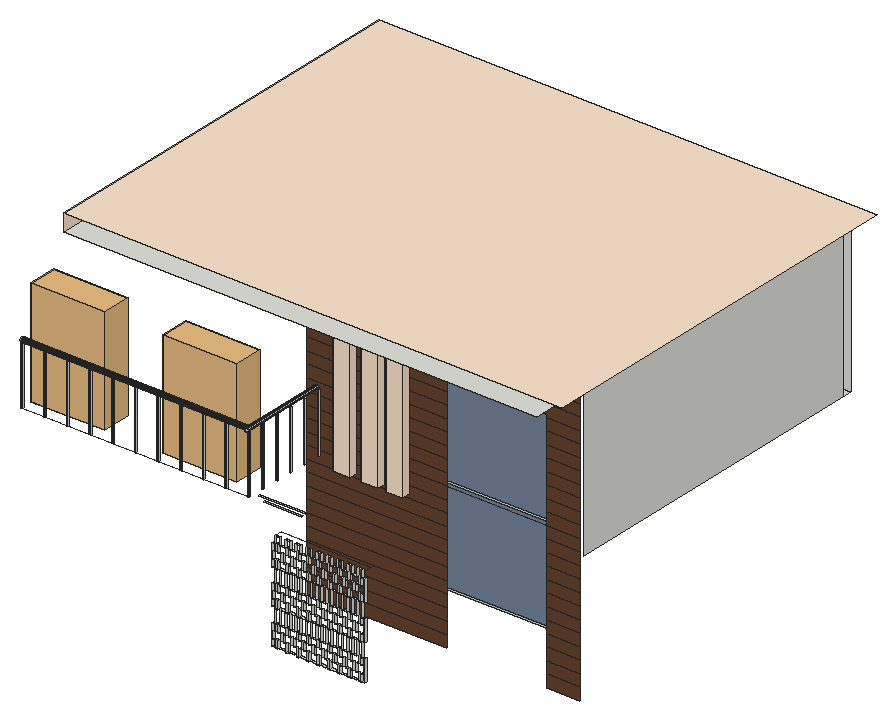
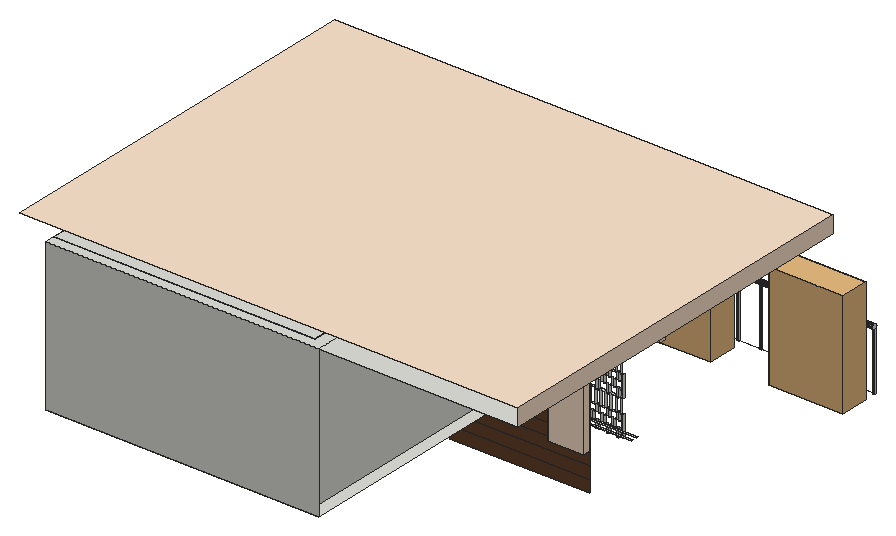
# SketchUp Ruby script. Lengths in inches.
U = 1.inch
M = Sketchup.active_model
def pt(a) = Geom::Point3d.new(a.map { |v| v * U })
def face(e, loops, mat)
  f = e.add_face(loops[0].map { |a| pt(a) })
  loops[1..].each { |l| e.add_face(l.map { |a| pt(a) }).erase! }
  f.material = f.back_material = mat if mat
  f
end
# faces: each face lists its corners as indices into pts; further lists are holes
def faces(e, pts, list, mat = nil) = list.each { |f| face(e, (f[0].is_a?(Array) ? f : [f]).map { |l| l.map { |i| pts[i] } }, mat) }
# xy, xz, yz: faces in a plane at the given z, y or x. An outline is a flat list of corners, or four numbers for a rectangle; further outlines are holes
def ring(l) = l.size == 4 ? [[l[0], l[1]], [l[2], l[1]], [l[2], l[3]], [l[0], l[3]]] : l.each_slice(2).to_a
def flat(e, list, mat, &to3) = list.each { |f| face(e, (f[0].is_a?(Array) ? f : [f]).map { |l| ring(l).map { |u, v| to3.(u, v) } }, mat) }
def xy(e, z, list, mat = nil) = flat(e, list, mat) { |x, y| [x, y, z] }
def xz(e, y, list, mat = nil) = flat(e, list, mat) { |x, z| [x, y, z] }
def yz(e, x, list, mat = nil) = flat(e, list, mat) { |y, z| [x, y, z] }
def lines(e, pts, list) = list.each { |a, b| e.add_line(pt(pts[a]), pt(pts[b])) }
# prism: a flat outline (further loops are holes) pulled along v
def prism(e, loops, v, mat = nil)
  f = face(e, loops, mat); d = Geom::Vector3d.new(v.map { |x| x * U })
  f.pushpull(f.normal.samedirection?(d) ? d.length : -d.length)
end
def box(e, o, s, mat = nil) = prism(e, [[o, [o[0] + s[0], o[1], o[2]], [o[0] + s[0], o[1] + s[1], o[2]], [o[0], o[1] + s[1], o[2]]]], [0, 0, s[2]], mat)
def at(x, y, z, deg = 0) = Geom::Transformation.translation(pt([x, y, z])) * Geom::Transformation.rotation(ORIGIN, Z_AXIS, deg.degrees)
def axes(o, x, y, z) = Geom::Transformation.new([*x, 0, *y, 0, *z, 0, *pt(o).to_a, 1])
def part(name) = M.definitions.add(name)
# library, detail: a bought-in or finely detailed component or shape, given as its bounding box
def library(name, o, s) = part(name).tap { |d| box(d.entities, o, s) }
def detail(e, o, s) = box(e.add_group.entities, o, s)
def put(e, d, t, mat = nil) = e.add_instance(d, t).tap { |i| i.material = mat if mat }
def group(e, t, mat = nil) = e.add_group.tap { |g| g.transformation = t; g.material = mat if mat }.entities
root = M.entities
M.materials.add("C01_Vanilla_Cream").color = [255, 230, 206]
M.materials.add("Glass_Mirror_01").color = [119, 135, 160]
M.materials.add("Wood_Veneer_15_1K").color = [103, 69, 45]
c1 = library("Group_2",[-1.28,-0.39,0],[21.22,20.51,48.44])
xy(root,373.98,[[283.14,137.21,284.89,138.74],[290.55,137.21,292.3,138.74],[297.96,137.21,299.71,138.74],[305.37,137.21,307.12,138.74],[312.78,137.21,314.53,138.74],
  [320.1875,137.21,321.94,138.74],[327.6,137.21,329.35,138.74],[335.01,137.21,336.76,138.74],[342.42,137.21,344.17,138.74]])
xy(root,374.38,[[280.31,137.21,282.27,138.74],[285.76,137.21,289.68,138.74],[293.17,137.21,297.09,138.74],[300.58,137.21,304.5,138.74],[307.99,137.21,311.91,138.74],
  [315.4,137.21,319.32,138.74],[322.81,137.21,326.73,138.74],[330.22,137.21,334.14,138.74],[337.63,137.21,341.55,138.74],[345.04,137.21,347,138.74]])
xy(root,379.25,[[281.18,137.21,283.14,138.74],[284.89,137.21,286.85,138.74],[288.59,137.21,290.55,138.74],[292.3,137.21,294.26,138.74],[296,137.21,297.96,138.74],
  [299.71,137.21,301.67,138.74],[303.41,137.21,305.37,138.74],[307.12,137.21,309.08,138.74],[310.82,137.21,312.78,138.74],[314.53,137.21,316.49,138.74],
  [318.23,137.21,320.1875,138.74],[321.94,137.21,323.9,138.74],[325.64,137.21,327.6,138.74],[329.35,137.21,331.31,138.74],[333.05,137.21,335.01,138.74],
  [336.76,137.21,338.72,138.74],[340.46,137.21,342.42,138.74],[344.17,137.21,346.13,138.74]])
xy(root,384.61,[[281.18,137.21,283.14,138.74],[284.89,137.21,286.85,138.74],[288.59,137.21,290.55,138.74],[292.3,137.21,294.26,138.74],[296,137.21,297.96,138.74],
  [299.71,137.21,301.67,138.74],[303.41,137.21,305.37,138.74],[307.12,137.21,309.08,138.74],[310.82,137.21,312.78,138.74],[314.53,137.21,316.49,138.74],
  [318.23,137.21,320.1875,138.74],[321.94,137.21,323.9,138.74],[325.64,137.21,327.6,138.74],[329.35,137.21,331.31,138.74],[333.05,137.21,335.01,138.74],
  [336.76,137.21,338.72,138.74],[340.46,137.21,342.42,138.74],[344.17,137.21,346.13,138.74]])
xy(root,389.47,[[280.31,137.21,282.27,138.74],[285.76,137.21,289.68,138.74],[293.17,137.21,297.09,138.74],[300.58,137.21,304.5,138.74],[307.99,137.21,311.91,138.74],
  [315.4,137.21,319.32,138.74],[322.81,137.21,326.73,138.74],[330.22,137.21,334.14,138.74],[337.63,137.21,341.55,138.74],[345.04,137.21,347,138.74]])
xy(root,389.875,[[283.14,137.21,284.89,138.74],[290.55,137.21,292.3,138.74],[297.96,137.21,299.71,138.74],[305.37,137.21,307.12,138.74],[312.78,137.21,314.53,138.74],
  [320.1875,137.21,321.94,138.74],[327.6,137.21,329.35,138.74],[335.01,137.21,336.76,138.74],[342.42,137.21,344.17,138.74]])
xy(root,399.61,[[283.14,137.21,284.89,138.74],[290.55,137.21,292.3,138.74],[297.96,137.21,299.71,138.74],[305.37,137.21,307.12,138.74],[312.78,137.21,314.53,138.74],
  [320.1875,137.21,321.94,138.74],[327.6,137.21,329.35,138.74],[335.01,137.21,336.76,138.74],[342.42,137.21,344.17,138.74]])
xy(root,400.01,[[280.31,137.21,282.27,138.74],[285.76,137.21,289.68,138.74],[293.17,137.21,297.09,138.74],[300.58,137.21,304.5,138.74],[307.99,137.21,311.91,138.74],
  [315.4,137.21,319.32,138.74],[322.81,137.21,326.73,138.74],[330.22,137.21,334.14,138.74],[337.63,137.21,341.55,138.74],[345.04,137.21,347,138.74]])
xy(root,404.88,[[281.18,137.21,283.14,138.74],[284.89,137.21,286.85,138.74],[288.59,137.21,290.55,138.74],[292.3,137.21,294.26,138.74],[296,137.21,297.96,138.74],
  [299.71,137.21,301.67,138.74],[303.41,137.21,305.37,138.74],[307.12,137.21,309.08,138.74],[310.82,137.21,312.78,138.74],[314.53,137.21,316.49,138.74],
  [318.23,137.21,320.1875,138.74],[321.94,137.21,323.9,138.74],[325.64,137.21,327.6,138.74],[329.35,137.21,331.31,138.74],[333.05,137.21,335.01,138.74],
  [336.76,137.21,338.72,138.74],[340.46,137.21,342.42,138.74],[344.17,137.21,346.13,138.74]])
xy(root,410.24,[[281.18,137.21,283.14,138.74],[284.89,137.21,286.85,138.74],[288.59,137.21,290.55,138.74],[292.3,137.21,294.26,138.74],[296,137.21,297.96,138.74],
  [299.71,137.21,301.67,138.74],[303.41,137.21,305.37,138.74],[307.12,137.21,309.08,138.74],[310.82,137.21,312.78,138.74],[314.53,137.21,316.49,138.74],
  [318.23,137.21,320.1875,138.74],[321.94,137.21,323.9,138.74],[325.64,137.21,327.6,138.74],[329.35,137.21,331.31,138.74],[333.05,137.21,335.01,138.74],
  [336.76,137.21,338.72,138.74],[340.46,137.21,342.42,138.74],[344.17,137.21,346.13,138.74]])
xy(root,415.1,[[280.31,137.21,282.27,138.74],[285.76,137.21,289.68,138.74],[293.17,137.21,297.09,138.74],[300.58,137.21,304.5,138.74],[307.99,137.21,311.91,138.74],
  [315.4,137.21,319.32,138.74],[322.81,137.21,326.73,138.74],[330.22,137.21,334.14,138.74],[337.63,137.21,341.55,138.74],[345.04,137.21,347,138.74]])
xy(root,415.5,[[283.14,137.21,284.89,138.74],[290.55,137.21,292.3,138.74],[297.96,137.21,299.71,138.74],[305.37,137.21,307.12,138.74],[312.78,137.21,314.53,138.74],
  [320.1875,137.21,321.94,138.74],[327.6,137.21,329.35,138.74],[335.01,137.21,336.76,138.74],[342.42,137.21,344.17,138.74]])
xy(root,425.24,[[283.14,137.21,284.89,138.74],[290.55,137.21,292.3,138.74],[297.96,137.21,299.71,138.74],[305.37,137.21,307.12,138.74],[312.78,137.21,314.53,138.74],
  [320.1875,137.21,321.94,138.74],[327.6,137.21,329.35,138.74],[335.01,137.21,336.76,138.74],[342.42,137.21,344.17,138.74]])
xy(root,425.64,[[280.31,137.21,282.27,138.74],[285.76,137.21,289.68,138.74],[293.17,137.21,297.09,138.74],[300.58,137.21,304.5,138.74],[307.99,137.21,311.91,138.74],
  [315.4,137.21,319.32,138.74],[322.81,137.21,326.73,138.74],[330.22,137.21,334.14,138.74],[337.63,137.21,341.55,138.74],[345.04,137.21,347,138.74]])
xy(root,430.51,[[281.18,137.21,283.14,138.74],[284.89,137.21,286.85,138.74],[288.59,137.21,290.55,138.74],[292.3,137.21,294.26,138.74],[296,137.21,297.96,138.74],
  [299.71,137.21,301.67,138.74],[303.41,137.21,305.37,138.74],[307.12,137.21,309.08,138.74],[310.82,137.21,312.78,138.74],[314.53,137.21,316.49,138.74],
  [318.23,137.21,320.1875,138.74],[321.94,137.21,323.9,138.74],[325.64,137.21,327.6,138.74],[329.35,137.21,331.31,138.74],[333.05,137.21,335.01,138.74],
  [336.76,137.21,338.72,138.74],[340.46,137.21,342.42,138.74],[344.17,137.21,346.13,138.74]])
xy(root,435.86,[[281.18,137.21,283.14,138.74],[284.89,137.21,286.85,138.74],[288.59,137.21,290.55,138.74],[292.3,137.21,294.26,138.74],[296,137.21,297.96,138.74],
  [299.71,137.21,301.67,138.74],[303.41,137.21,305.37,138.74],[307.12,137.21,309.08,138.74],[310.82,137.21,312.78,138.74],[314.53,137.21,316.49,138.74],
  [318.23,137.21,320.1875,138.74],[321.94,137.21,323.9,138.74],[325.64,137.21,327.6,138.74],[329.35,137.21,331.31,138.74],[333.05,137.21,335.01,138.74],
  [336.76,137.21,338.72,138.74],[340.46,137.21,342.42,138.74],[344.17,137.21,346.13,138.74]])
xy(root,440.73,[[280.31,137.21,282.27,138.74],[285.76,137.21,289.68,138.74],[293.17,137.21,297.09,138.74],[300.58,137.21,304.5,138.74],[307.99,137.21,311.91,138.74],
  [315.4,137.21,319.32,138.74],[322.81,137.21,326.73,138.74],[330.22,137.21,334.14,138.74],[337.63,137.21,341.55,138.74],[345.04,137.21,347,138.74]])
xy(root,441.13,[[283.14,137.21,284.89,138.74],[290.55,137.21,292.3,138.74],[297.96,137.21,299.71,138.74],[305.37,137.21,307.12,138.74],[312.78,137.21,314.53,138.74],
  [320.1875,137.21,321.94,138.74],[327.6,137.21,329.35,138.74],[335.01,137.21,336.76,138.74],[342.42,137.21,344.17,138.74]])
xy(root,446,[[282.27,137.21,285.76,138.74],[289.68,137.21,293.17,138.74],[297.09,137.21,300.58,138.74],[304.5,137.21,307.99,138.74],[311.91,137.21,315.4,138.74],
  [319.32,137.21,322.81,138.74],[326.73,137.21,330.22,138.74],[334.14,137.21,337.63,138.74],[341.55,137.21,345.04,138.74]])
xy(root,465,[[263.64,136.51,264.8,137.09],[282.61,189.3,294.64,194.88],[302.46,189.3,314.49,194.88],[320.42,189.3,332.45,194.88],[256.9,201,256.9,441,453,441,453,433.71,265.5,433.71,265.5,201],
  [185.32,287.91,211.07,293.09]])
xy(root,507.13,[[263.64,136.51,264.8,137.09]])
xy(root,549,[[357,198,429,199.5]])
xy(root,555.9375,[[130.74,287.91,185.32,293.09],[211.07,287.91,256.9,293.09]],"C01_Vanilla_Cream")
xy(root,573,[[[114,158.82,114,441,256.9,441,256.9,198,453,198,453,158.82],[320.42,189.3,332.45,194.88],[302.46,189.3,314.49,194.88],[282.61,189.3,294.64,194.88]],[256.9,198,256.9,441,453,441,453,433.71,265.5,433.71,265.5,201,453,201,453,198],[265.5,201,453,433.71]])
xy(root,579.87,[[130.74,287.91,256.9,293.09]])
xy(root,585,[[114,158.82,471,441]],"C01_Vanilla_Cream")
xz(root,135.29,[[263.64,507.13,264.01,507.18,264.36,507.32,264.66,507.55,264.89,507.85,265.04,508.2,265.09,508.58,265.04,508.96,264.89,509.31,264.66,509.61,264.36,509.84,264.01,509.98,263.64,510.03,263.26,509.98,262.91,509.84,262.61,509.61,262.38,509.31,262.27,509.05,262.24,508.96,262.1875,508.58,262.24,508.2,262.38,507.85,262.61,507.55,262.91,507.32,263.26,507.18]])
xz(root,136.51,[[100.9,465,102.07,507.13],[117.18,465,118.34,507.13],[133.45,465,134.62,507.13],[149.72,465,150.89,507.13],[166,465,167.16,507.13],
  [182.27,465,183.44,507.13],[198.54,465,199.71,507.13],[214.82,465,215.98,507.13],[231.09,465,232.26,507.13],[247.36,465,248.53,507.13],
  [263.64,465,264.8,507.13]])
xz(root,137.09,[[100.9,465,102.07,507.13],[117.18,465,118.34,507.13],[133.45,465,134.62,507.13],[149.72,465,150.89,507.13],[166,465,167.16,507.13],
  [182.27,465,183.44,507.13],[198.54,465,199.71,507.13],[214.82,465,215.98,507.13],[231.09,465,232.26,507.13],[247.36,465,248.53,507.13],
  [263.64,465,264.8,507.13]])
xz(root,148.6875,[[263.9,465,265.0625,507.13]])
xz(root,149.27,[[263.9,465,265.0625,507.13]])
xz(root,160.87,[[264.16,465,265.32,507.13]])
xz(root,161.46,[[264.16,465,265.32,507.13]])
xz(root,173.05,[[264.42,465,265.59,507.13]])
xz(root,173.64,[[264.42,465,265.59,507.13]])
xz(root,185.23,[[264.68,465,265.85,507.13]])
xz(root,185.82,[[264.68,465,265.85,507.13]])
xz(root,189.3,[[282.61,465,294.64,573],[302.46,465,314.49,573],[320.42,465,332.45,573]],"C01_Vanilla_Cream")
xz(root,194.88,[[282.61,465,294.64,573],[302.46,465,314.49,573],[320.42,465,332.45,573]])
xz(root,197.41,[[264.94,465,266.11,507.13]])
xz(root,198,[[264.94,494.88,266.11,503.56]])
xz(root,198,[[256.9,373.36,357,382.04],[429,373.36,453,382.04],[256.9,382.04,357,390.72],[429,382.04,453,390.72],[256.9,390.72,357,399.4],
  [429,390.72,453,399.4],[256.9,399.4,357,408.08],[429,399.4,453,408.08],[256.9,408.08,357,416.76],[429,408.08,453,416.76],
  [256.9,416.76,357,425.44],[429,416.76,453,425.44],[256.9,425.44,357,434.12],[429,425.44,453,434.12],[256.9,434.12,357,442.8],
  [429,434.12,453,442.8],[256.9,442.8,357,451.48],[429,442.8,453,451.48],[256.9,451.48,357,460.16],[429,451.48,453,460.16],
  [256.9,460.16,357,460.16,357,468.84,266.11,468.84,266.11,465,264.94,465,264.94,468.84,256.9,468.84],[429,460.16,453,468.84],[264.94,465,266.11,468.84],[256.9,468.84,264.94,477.52],[264.94,468.84,266.11,477.52],
  [266.11,468.84,357,477.52],[429,468.84,453,477.52],[256.9,477.52,264.94,486.2],[264.94,477.52,266.11,486.2],[266.11,477.52,357,486.2],
  [429,477.52,453,486.2],[256.9,486.2,264.94,494.88],[264.94,486.2,266.11,494.88],[266.11,486.2,357,494.88],[429,486.2,453,494.88],
  [256.9,494.88,264.94,503.56],[266.11,494.88,357,503.56],[429,494.88,453,503.56],[[256.9,503.56,264.94,503.56,264.94,507.13,266.11,507.13,266.11,503.56,357,503.56,357,512.24,256.9,512.24],[263.64,507.13,263.26,507.18,262.91,507.32,262.61,507.55,262.38,507.85,262.24,508.2,262.1875,508.58,262.24,508.96,262.38,509.31,262.61,509.61,262.91,509.84,263.26,509.98,263.64,510.03,264.01,509.98,264.36,509.84,264.66,509.61,264.89,509.31,265.04,508.96,265.09,508.58,265.04,508.2,264.89,507.85,264.66,507.55,264.36,507.32,264.01,507.18]],[264.94,503.56,266.11,507.13],
  [429,503.56,453,512.24],[256.9,512.24,357,520.92],[429,512.24,453,520.92],[256.9,520.92,357,529.6],[429,520.92,453,529.6],
  [256.9,529.6,357,538.28],[429,529.6,453,538.28],[256.9,538.28,357,546.96],[429,538.28,453,546.96],[256.9,546.96,357,546.96,357,549,429,549,429,546.96,453,546.96,453,555.64,256.9,555.64],
  [256.9,555.64,453,564.32],[256.9,564.32,453,573]],"Wood_Veneer_15_1K")
xz(root,199.5,[[357,410.35,429,411.35],[357,479.17,429,480.17],[357,548,429,549]])
xz(root,199.5,[[357,411.35,429,479.17],[357,480.17,429,548]],"Glass_Mirror_01")
xz(root,287.91,[[185.32,465,211.07,465,211.07,555.9375,256.9,555.9375,256.9,579.87,130.74,579.87,130.74,555.9375,185.32,555.9375]],"C01_Vanilla_Cream")
xz(root,293.09,[[185.32,465,185.32,555.9375,130.74,555.9375,130.74,579.87,256.9,579.87,256.9,555.9375,211.07,555.9375,211.07,465]],"C01_Vanilla_Cream")
xz(root,433.71,[[265.5,465,453,573]])
xz(root,441,[[256.9,465,453,573]])
yz(root,100.9,[[136.51,465,137.09,507.13],[137.24,507.1,137.09,507.13,136.86,507.17,136.51,507.34,136.22,507.6,136,507.91,135.875,508.28,135.85,508.67,135.92,509.05,136.09,509.39,136.34,509.6875,136.66,509.9,137.03,510.03,137.41,510.06,137.79,509.99,138.14,509.82,138.43,509.56,138.65,509.24,138.78,508.88,138.8,508.49,138.73,508.11,138.5625,507.77,138.3125,507.47,137.99,507.26,137.625,507.13]])
yz(root,102.07,[[136.51,465,137.09,507.13]])
yz(root,114,[[158.82,573,441,585]],"C01_Vanilla_Cream")
yz(root,117.18,[[136.51,465,137.09,507.13]])
yz(root,118.34,[[136.51,465,137.09,507.13]])
yz(root,130.74,[[287.91,555.9375,293.09,579.87]],"C01_Vanilla_Cream")
yz(root,133.45,[[136.51,465,137.09,507.13]])
yz(root,134.62,[[136.51,465,137.09,507.13]])
yz(root,149.72,[[136.51,465,137.09,507.13]])
yz(root,150.89,[[136.51,465,137.09,507.13]])
yz(root,166,[[136.51,465,137.09,507.13]])
yz(root,167.16,[[136.51,465,137.09,507.13]])
yz(root,182.27,[[136.51,465,137.09,507.13]])
yz(root,183.44,[[136.51,465,137.09,507.13]])
yz(root,185.32,[[287.91,465,293.09,555.9375]],"C01_Vanilla_Cream")
yz(root,198.54,[[136.51,465,137.09,507.13]])
yz(root,199.71,[[136.51,465,137.09,507.13]])
yz(root,211.07,[[287.91,465,293.09,555.9375]],"C01_Vanilla_Cream")
yz(root,214.82,[[136.51,465,137.09,507.13]])
yz(root,215.98,[[136.51,465,137.09,507.13]])
yz(root,231.09,[[136.51,465,137.09,507.13]])
yz(root,232.26,[[136.51,465,137.09,507.13]])
yz(root,247.36,[[136.51,465,137.09,507.13]])
yz(root,248.53,[[136.51,465,137.09,507.13]])
yz(root,256.9,[[287.91,555.9375,293.09,573],[287.91,573,293.09,579.87]])
yz(root,263.64,[[136.51,465,137.09,507.13],[137.24,507.1,137.625,507.13,137.09,507.13],[137.09,507.13,137.625,507.13,137.99,507.26,138.3125,507.47,138.5625,507.77,138.73,508.11,138.8,508.49,138.8,508.58,138.78,508.88,138.65,509.24,138.43,509.56,138.14,509.82,137.79,509.99,137.56,510.03,137.03,510.03,136.66,509.9,136.34,509.6875,136.09,509.39,135.92,509.05,135.85,508.67,135.875,508.28,136,507.91,136.22,507.6,136.51,507.34,136.86,507.17],[137.03,510.03,137.56,510.03,137.41,510.06]])
yz(root,263.9,[[148.6875,465,149.27,507.13]])
yz(root,264.16,[[160.87,465,161.46,507.13]])
yz(root,264.42,[[173.05,465,173.64,507.13]])
yz(root,264.68,[[185.23,465,185.82,507.13]])
yz(root,264.8,[[136.51,465,137.09,507.13]])
yz(root,264.94,[[197.41,465,198,507.13]])
yz(root,265.0625,[[148.6875,465,149.27,507.13]])
yz(root,265.32,[[160.87,465,161.46,507.13]])
yz(root,265.5,[[201,465,433.71,573]])
yz(root,265.59,[[173.05,465,173.64,507.13]])
yz(root,265.85,[[185.23,465,185.82,507.13]])
yz(root,266.11,[[197.41,465,198,507.13]])
yz(root,280.31,[[137.21,374.38,138.74,389.47],[137.21,400.01,138.74,415.1],[137.21,425.64,138.74,440.73]])
yz(root,281.18,[[137.21,379.25,138.74,384.61],[137.21,404.88,138.74,410.24],[137.21,430.51,138.74,435.86]])
yz(root,282.27,[[137.21,389.47,138.74,400.01],[137.21,415.1,138.74,425.64],[137.21,440.73,138.74,446]])
yz(root,282.61,[[189.3,465,194.88,573]],"C01_Vanilla_Cream")
yz(root,283.14,[[137.21,373.98,138.74,379.25],[137.21,384.61,138.74,389.875],[137.21,399.61,138.74,404.88],[137.21,410.24,138.74,415.5],[137.21,425.24,138.74,430.51],
  [137.21,435.86,138.74,441.13]])
yz(root,284.89,[[137.21,373.98,138.74,379.25],[137.21,384.61,138.74,389.875],[137.21,399.61,138.74,404.88],[137.21,410.24,138.74,415.5],[137.21,425.24,138.74,430.51],
  [137.21,435.86,138.74,441.13]])
yz(root,285.76,[[137.21,389.47,138.74,400.01],[137.21,415.1,138.74,425.64],[137.21,440.73,138.74,446]])
yz(root,286.85,[[137.21,379.25,138.74,384.61],[137.21,404.88,138.74,410.24],[137.21,430.51,138.74,435.86]])
yz(root,288.59,[[137.21,379.25,138.74,384.61],[137.21,404.88,138.74,410.24],[137.21,430.51,138.74,435.86]])
yz(root,289.68,[[137.21,389.47,138.74,400.01],[137.21,415.1,138.74,425.64],[137.21,440.73,138.74,446]])
yz(root,290.55,[[137.21,373.98,138.74,379.25],[137.21,384.61,138.74,389.875],[137.21,399.61,138.74,404.88],[137.21,410.24,138.74,415.5],[137.21,425.24,138.74,430.51],
  [137.21,435.86,138.74,441.13]])
yz(root,292.3,[[137.21,373.98,138.74,379.25],[137.21,384.61,138.74,389.875],[137.21,399.61,138.74,404.88],[137.21,410.24,138.74,415.5],[137.21,425.24,138.74,430.51],
  [137.21,435.86,138.74,441.13]])
yz(root,293.17,[[137.21,389.47,138.74,400.01],[137.21,415.1,138.74,425.64],[137.21,440.73,138.74,446]])
yz(root,294.26,[[137.21,379.25,138.74,384.61],[137.21,404.88,138.74,410.24],[137.21,430.51,138.74,435.86]])
yz(root,294.64,[[189.3,465,194.88,573]],"C01_Vanilla_Cream")
yz(root,296,[[137.21,379.25,138.74,384.61],[137.21,404.88,138.74,410.24],[137.21,430.51,138.74,435.86]])
yz(root,297.09,[[137.21,389.47,138.74,400.01],[137.21,415.1,138.74,425.64],[137.21,440.73,138.74,446]])
yz(root,297.96,[[137.21,373.98,138.74,379.25],[137.21,384.61,138.74,389.875],[137.21,399.61,138.74,404.88],[137.21,410.24,138.74,415.5],[137.21,425.24,138.74,430.51],
  [137.21,435.86,138.74,441.13]])
yz(root,299.71,[[137.21,373.98,138.74,379.25],[137.21,384.61,138.74,389.875],[137.21,399.61,138.74,404.88],[137.21,410.24,138.74,415.5],[137.21,425.24,138.74,430.51],
  [137.21,435.86,138.74,441.13]])
yz(root,300.58,[[137.21,389.47,138.74,400.01],[137.21,415.1,138.74,425.64],[137.21,440.73,138.74,446]])
yz(root,301.67,[[137.21,379.25,138.74,384.61],[137.21,404.88,138.74,410.24],[137.21,430.51,138.74,435.86]])
yz(root,302.46,[[189.3,465,194.88,573]],"C01_Vanilla_Cream")
yz(root,303.41,[[137.21,379.25,138.74,384.61],[137.21,404.88,138.74,410.24],[137.21,430.51,138.74,435.86]])
yz(root,304.5,[[137.21,389.47,138.74,400.01],[137.21,415.1,138.74,425.64],[137.21,440.73,138.74,446]])
yz(root,305.37,[[137.21,373.98,138.74,379.25],[137.21,384.61,138.74,389.875],[137.21,399.61,138.74,404.88],[137.21,410.24,138.74,415.5],[137.21,425.24,138.74,430.51],
  [137.21,435.86,138.74,441.13]])
yz(root,307.12,[[137.21,373.98,138.74,379.25],[137.21,384.61,138.74,389.875],[137.21,399.61,138.74,404.88],[137.21,410.24,138.74,415.5],[137.21,425.24,138.74,430.51],
  [137.21,435.86,138.74,441.13]])
yz(root,307.99,[[137.21,389.47,138.74,400.01],[137.21,415.1,138.74,425.64],[137.21,440.73,138.74,446]])
yz(root,309.08,[[137.21,379.25,138.74,384.61],[137.21,404.88,138.74,410.24],[137.21,430.51,138.74,435.86]])
yz(root,310.82,[[137.21,379.25,138.74,384.61],[137.21,404.88,138.74,410.24],[137.21,430.51,138.74,435.86]])
yz(root,311.91,[[137.21,389.47,138.74,400.01],[137.21,415.1,138.74,425.64],[137.21,440.73,138.74,446]])
yz(root,312.78,[[137.21,373.98,138.74,379.25],[137.21,384.61,138.74,389.875],[137.21,399.61,138.74,404.88],[137.21,410.24,138.74,415.5],[137.21,425.24,138.74,430.51],
  [137.21,435.86,138.74,441.13]])
yz(root,314.49,[[189.3,465,194.88,573]],"C01_Vanilla_Cream")
yz(root,314.53,[[137.21,373.98,138.74,379.25],[137.21,384.61,138.74,389.875],[137.21,399.61,138.74,404.88],[137.21,410.24,138.74,415.5],[137.21,425.24,138.74,430.51],
  [137.21,435.86,138.74,441.13]])
yz(root,315.4,[[137.21,389.47,138.74,400.01],[137.21,415.1,138.74,425.64],[137.21,440.73,138.74,446]])
yz(root,316.49,[[137.21,379.25,138.74,384.61],[137.21,404.88,138.74,410.24],[137.21,430.51,138.74,435.86]])
yz(root,318.23,[[137.21,379.25,138.74,384.61],[137.21,404.88,138.74,410.24],[137.21,430.51,138.74,435.86]])
yz(root,319.32,[[137.21,389.47,138.74,400.01],[137.21,415.1,138.74,425.64],[137.21,440.73,138.74,446]])
yz(root,320.1875,[[137.21,373.98,138.74,379.25],[137.21,384.61,138.74,389.875],[137.21,399.61,138.74,404.88],[137.21,410.24,138.74,415.5],[137.21,425.24,138.74,430.51],
  [137.21,435.86,138.74,441.13]])
yz(root,320.42,[[189.3,465,194.88,573]],"C01_Vanilla_Cream")
yz(root,321.94,[[137.21,373.98,138.74,379.25],[137.21,384.61,138.74,389.875],[137.21,399.61,138.74,404.88],[137.21,410.24,138.74,415.5],[137.21,425.24,138.74,430.51],
  [137.21,435.86,138.74,441.13]])
yz(root,322.81,[[137.21,389.47,138.74,400.01],[137.21,415.1,138.74,425.64],[137.21,440.73,138.74,446]])
yz(root,323.9,[[137.21,379.25,138.74,384.61],[137.21,404.88,138.74,410.24],[137.21,430.51,138.74,435.86]])
yz(root,325.64,[[137.21,379.25,138.74,384.61],[137.21,404.88,138.74,410.24],[137.21,430.51,138.74,435.86]])
yz(root,326.73,[[137.21,389.47,138.74,400.01],[137.21,415.1,138.74,425.64],[137.21,440.73,138.74,446]])
yz(root,327.6,[[137.21,373.98,138.74,379.25],[137.21,384.61,138.74,389.875],[137.21,399.61,138.74,404.88],[137.21,410.24,138.74,415.5],[137.21,425.24,138.74,430.51],
  [137.21,435.86,138.74,441.13]])
yz(root,329.35,[[137.21,373.98,138.74,379.25],[137.21,384.61,138.74,389.875],[137.21,399.61,138.74,404.88],[137.21,410.24,138.74,415.5],[137.21,425.24,138.74,430.51],
  [137.21,435.86,138.74,441.13]])
yz(root,330.22,[[137.21,389.47,138.74,400.01],[137.21,415.1,138.74,425.64],[137.21,440.73,138.74,446]])
yz(root,331.31,[[137.21,379.25,138.74,384.61],[137.21,404.88,138.74,410.24],[137.21,430.51,138.74,435.86]])
yz(root,332.45,[[189.3,465,194.88,573]],"C01_Vanilla_Cream")
yz(root,333.05,[[137.21,379.25,138.74,384.61],[137.21,404.88,138.74,410.24],[137.21,430.51,138.74,435.86]])
yz(root,334.14,[[137.21,389.47,138.74,400.01],[137.21,415.1,138.74,425.64],[137.21,440.73,138.74,446]])
yz(root,335.01,[[137.21,373.98,138.74,379.25],[137.21,384.61,138.74,389.875],[137.21,399.61,138.74,404.88],[137.21,410.24,138.74,415.5],[137.21,425.24,138.74,430.51],
  [137.21,435.86,138.74,441.13]])
yz(root,336.76,[[137.21,373.98,138.74,379.25],[137.21,384.61,138.74,389.875],[137.21,399.61,138.74,404.88],[137.21,410.24,138.74,415.5],[137.21,425.24,138.74,430.51],
  [137.21,435.86,138.74,441.13]])
yz(root,337.63,[[137.21,389.47,138.74,400.01],[137.21,415.1,138.74,425.64],[137.21,440.73,138.74,446]])
yz(root,338.72,[[137.21,379.25,138.74,384.61],[137.21,404.88,138.74,410.24],[137.21,430.51,138.74,435.86]])
yz(root,340.46,[[137.21,379.25,138.74,384.61],[137.21,404.88,138.74,410.24],[137.21,430.51,138.74,435.86]])
yz(root,341.55,[[137.21,389.47,138.74,400.01],[137.21,415.1,138.74,425.64],[137.21,440.73,138.74,446]])
yz(root,342.42,[[137.21,373.98,138.74,379.25],[137.21,384.61,138.74,389.875],[137.21,399.61,138.74,404.88],[137.21,410.24,138.74,415.5],[137.21,425.24,138.74,430.51],
  [137.21,435.86,138.74,441.13]])
yz(root,344.17,[[137.21,373.98,138.74,379.25],[137.21,384.61,138.74,389.875],[137.21,399.61,138.74,404.88],[137.21,410.24,138.74,415.5],[137.21,425.24,138.74,430.51],
  [137.21,435.86,138.74,441.13]])
yz(root,345.04,[[137.21,389.47,138.74,400.01],[137.21,415.1,138.74,425.64],[137.21,440.73,138.74,446]])
yz(root,346.13,[[137.21,379.25,138.74,384.61],[137.21,404.88,138.74,410.24],[137.21,430.51,138.74,435.86]])
yz(root,347,[[137.21,374.38,138.74,389.47],[137.21,400.01,138.74,415.1],[137.21,425.64,138.74,440.73]])
yz(root,453,[[201,465,433.71,573]])
p = [[223.99,201.05,419.93],[251.32,201.05,419.93],[251.32,199.97,419.92],[223.99,199.97,419.92],[254.32,201,422.93],[220.99,201,422.93],
  [220.99,199.92,422.92],[254.32,199.92,422.92],[263.26,198,507.18],[263.64,198,507.13],[263.64,137.625,507.13],[263.64,137.09,507.13],
  [263.64,136.51,507.13],[263.64,136.34,507.13],[263.64,135.29,507.13],[263.26,135.29,507.18],[264.01,198,507.18],[264.01,135.29,507.18],
  [100.9,137.09,507.13],[100.9,137.24,507.1],[263.64,137.24,507.1],[263.64,136.86,507.17],[100.9,136.86,507.17],[100.9,137.625,507.13],
  [100.9,137.99,507.26],[263.64,137.99,507.26],[262.91,198,507.32],[262.91,135.29,507.32],[264.36,198,507.32],[264.36,135.29,507.32],
  [100.9,136.51,507.34],[263.64,136.51,507.34],[262.61,198,507.55],[262.61,135.29,507.55],[264.66,198,507.55],[264.66,135.29,507.55],
  [100.9,136.22,507.6],[263.64,136.22,507.6],[100.9,138.3125,507.47],[263.64,138.3125,507.47],[100.9,138.5625,507.77],[263.64,138.5625,507.77],
  [262.38,198,507.85],[262.38,135.29,507.85],[264.89,198,507.85],[264.89,135.29,507.85],[100.9,136,507.91],[263.64,136,507.91],
  [100.9,138.73,508.11],[263.64,138.73,508.11],[262.24,198,508.2],[262.24,135.29,508.2],[265.04,198,508.2],[265.04,135.29,508.2],
  [100.9,135.875,508.28],[263.64,135.875,508.28],[100.9,138.8,508.49],[263.64,138.8,508.49],[262.1875,198,508.58],[262.1875,135.29,508.58],
  [265.09,198,508.58],[265.09,135.29,508.58],[100.9,135.85,508.67],[263.64,135.85,508.67],[100.9,138.78,508.88],[263.64,138.78,508.88],
  [263.64,138.8,508.58],[262.24,198,508.96],[262.24,135.29,508.96],[265.04,198,508.96],[265.04,135.29,508.96],[100.9,135.92,509.05],
  [263.64,135.92,509.05],[262.27,135.92,509.05],[100.9,138.65,509.24],[263.64,138.65,509.24],[262.38,198,509.31],[262.27,135.29,509.05],
  [262.38,135.29,509.31],[264.89,198,509.31],[264.89,135.29,509.31],[100.9,136.09,509.39],[263.64,136.09,509.39],[100.9,138.43,509.56],
  [263.64,138.43,509.56],[262.61,198,509.61],[262.61,135.29,509.61],[264.66,198,509.61],[264.66,135.29,509.61],[100.9,136.34,509.6875],
  [263.64,136.34,509.6875],[262.91,198,509.84],[262.91,135.29,509.84],[264.36,198,509.84],[264.36,135.29,509.84],[100.9,138.14,509.82],
  [263.64,138.14,509.82],[100.9,136.66,509.9],[263.64,136.66,509.9],[263.26,198,509.98],[263.26,135.29,509.98],[264.01,198,509.98],
  [264.01,135.29,509.98],[100.9,137.79,509.99],[263.64,137.79,509.99],[100.9,137.03,510.03],[263.64,137.03,510.03],[263.64,198,510.03],
  [263.64,135.29,510.03],[263.64,137.56,510.03],[100.9,137.41,510.06],[263.64,137.41,510.06],[254.32,201,422],[254.32,201,422.9],
  [254.32,201,446],[256.9,201,446],[256.33,201,422],[357,198,477.52],[429,198,477.52],[282.16,143.21,446],
  [347,142.6875,446],[346.97,136.6875,446],[282.125,137.21,446],[265.5,201,446],[265.5,201,465],[263.64,137.33,508.58],
  [263.64,198,508.58],[263.64,136.51,465],[248.53,136.51,465],[103.62,136.51,465],[102.07,136.51,465],[247.36,136.51,465],
  [232.26,136.51,465],[231.09,136.51,465],[215.98,136.51,465],[214.82,136.51,465],[199.71,136.51,465],[198.54,136.51,465],
  [183.44,136.51,465],[182.27,136.51,465],[167.16,136.51,465],[166,136.51,465],[150.89,136.51,465],[149.72,136.51,465],
  [134.62,136.51,465],[133.45,136.51,465],[118.34,136.51,465],[117.18,136.51,465]]
faces(root,p,[[0,1,2,3],[4,5,6,7],[8,9,10,11,12,13,14,15],[9,16,17,14,13,12,11,10],[18,19,20,11,21,22],[19,23,10,20],[23,24,25,10],[26,8,15,27],
  [16,28,29,17],[30,22,21,31],[32,26,27,33],[28,34,35,29],[36,30,31,37],[24,38,39,25],[38,40,41,39],[42,32,33,43],
  [34,44,45,35],[46,36,37,47],[40,48,49,41],[50,42,43,51],[44,52,53,45],[54,46,47,55],[48,56,57,49],[58,50,51,59],
  [52,60,61,53],[62,54,55,63],[56,64,65,66,57],[67,58,59,68],[60,69,70,61],[71,62,63,72,73],[64,74,75,65],[76,67,68,77,78],
  [69,79,80,70],[81,71,73,72,82],[74,83,84,75],[85,76,78,86],[79,87,88,80],[89,81,82,90],[91,85,86,92],[87,93,94,88],
  [83,95,96,84],[97,89,90,98],[99,91,92,100],[93,101,102,94],[95,103,104,96],[105,97,98,106],[107,99,100,108,106,109],[101,107,109,106,108,102],
  [110,105,106,111],[103,110,111,109,104]])
lines(root,p,[[112,113],[114,115],[4,114],[116,112],[117,118],[119,120],[120,121],[119,122],[123,124],[125,66],[66,126],[73,77],
  [127,128],[129,130],[131,132],[133,134],[135,136],[137,138],[139,140],[141,142],[143,144],[145,146],[147,129]])
put(root,c1,axes([104.08,145.92,465],[2.485,0,0],[0,1,0],[0,0,1.57]))
put(root,c1,axes([198.83,145.92,465],[2.485,0,0],[0,1,0],[0,0,1.57]))
